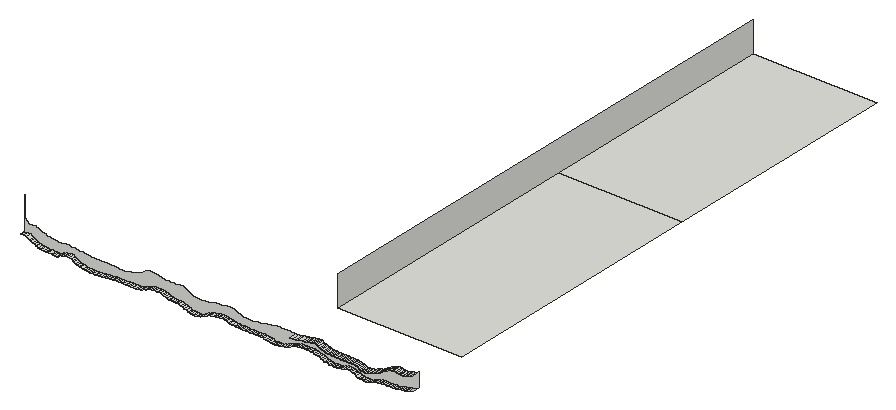
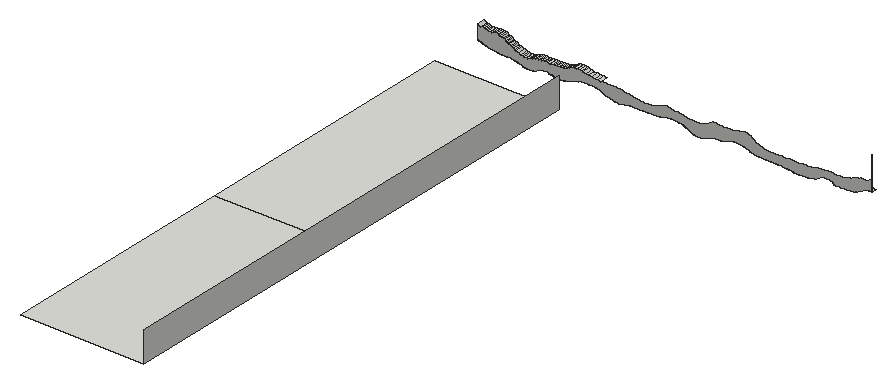
# SketchUp Ruby script. Lengths in inches.
U = 1.inch
M = Sketchup.active_model
def pt(a) = Geom::Point3d.new(a.map { |v| v * U })
def face(e, loops, mat)
  f = e.add_face(loops[0].map { |a| pt(a) })
  loops[1..].each { |l| e.add_face(l.map { |a| pt(a) }).erase! }
  f.material = f.back_material = mat if mat
  f
end
# faces: each face lists its corners as indices into pts; further lists are holes
def faces(e, pts, list, mat = nil) = list.each { |f| face(e, (f[0].is_a?(Array) ? f : [f]).map { |l| l.map { |i| pts[i] } }, mat) }
# xy, xz, yz: faces in a plane at the given z, y or x. An outline is a flat list of corners, or four numbers for a rectangle; further outlines are holes
def ring(l) = l.size == 4 ? [[l[0], l[1]], [l[2], l[1]], [l[2], l[3]], [l[0], l[3]]] : l.each_slice(2).to_a
def flat(e, list, mat, &to3) = list.each { |f| face(e, (f[0].is_a?(Array) ? f : [f]).map { |l| ring(l).map { |u, v| to3.(u, v) } }, mat) }
def xy(e, z, list, mat = nil) = flat(e, list, mat) { |x, y| [x, y, z] }
def xz(e, y, list, mat = nil) = flat(e, list, mat) { |x, z| [x, y, z] }
def yz(e, x, list, mat = nil) = flat(e, list, mat) { |y, z| [x, y, z] }
def lines(e, pts, list) = list.each { |a, b| e.add_line(pt(pts[a]), pt(pts[b])) }
# prism: a flat outline (further loops are holes) pulled along v
def prism(e, loops, v, mat = nil)
  f = face(e, loops, mat); d = Geom::Vector3d.new(v.map { |x| x * U })
  f.pushpull(f.normal.samedirection?(d) ? d.length : -d.length)
end
def box(e, o, s, mat = nil) = prism(e, [[o, [o[0] + s[0], o[1], o[2]], [o[0] + s[0], o[1] + s[1], o[2]], [o[0], o[1] + s[1], o[2]]]], [0, 0, s[2]], mat)
def at(x, y, z, deg = 0) = Geom::Transformation.translation(pt([x, y, z])) * Geom::Transformation.rotation(ORIGIN, Z_AXIS, deg.degrees)
def axes(o, x, y, z) = Geom::Transformation.new([*x, 0, *y, 0, *z, 0, *pt(o).to_a, 1])
def part(name) = M.definitions.add(name)
# library, detail: a bought-in or finely detailed component or shape, given as its bounding box
def library(name, o, s) = part(name).tap { |d| box(d.entities, o, s) }
def detail(e, o, s) = box(e.add_group.entities, o, s)
def put(e, d, t, mat = nil) = e.add_instance(d, t).tap { |i| i.material = mat if mat }
def group(e, t, mat = nil) = e.add_group.tap { |g| g.transformation = t; g.material = mat if mat }.entities
root = M.entities
xy(root,237.65,[[1160.83,566.68,1161.52,568.68],[1161.52,566.68,1162.14,568.68]])
xy(root,238.18,[[1254.78,566.68,1255.46,568.68]])
xy(root,238.33,[[1169.93,566.68,1170.48,568.68],[1170.48,566.68,1171.16,568.68]])
xy(root,238.34,[[1171.84,566.68,1172.77,568.68],[1172.77,566.68,1173.26,568.68],[1173.26,566.68,1174.02,568.68],[1174.02,566.68,1174.65,568.68],[1174.65,566.68,1175.4,568.68],
  [1175.4,566.68,1176.02,568.68],[1176.02,566.68,1176.79,568.68],[1176.79,566.68,1177.41,568.68]])
xy(root,238.62,[[1221.31,566.68,1222.08,568.68],[1222.08,566.68,1222.71,568.68],[1222.71,566.68,1223.47,568.68],[1223.47,566.68,1224.09,568.68],[1224.09,566.68,1224.94,568.68],
  [1224.94,566.68,1225.58,568.68],[1225.58,566.68,1226.2,568.68]])
xy(root,238.625,[[1219.89,566.68,1220.75,568.68]])
xy(root,238.89,[[1275.7,566.68,1276.38,568.68]])
xy(root,238.9,[[1277.14,566.68,1277.76,568.68],[1277.76,566.68,1278.53,568.68]])
xy(root,240.43,[[1243.98,566.68,1244.55,568.68]])
xy(root,241.52,[[1131.53,566.68,1131.59,568.68]])
xy(root,242.28,[[1261.8,565.74,1262.3125,568.68]])
xy(root,242.3,[[1260.04,565.74,1260.71,568.68]])
xy(root,242.33,[[1257.63,565.74,1258.21,568.68]])
xy(root,242.625,[[1237.14,589.83,1285.6,697.21],[1237.14,697.21,1285.6,792.52]])
xz(root,568.68,[[1200.45,236.98,1199.84,237.01,1199.15,237.04,1198.39,237.11,1197.7,237.2,1197.17,237.33,1196.5,237.68,1195.5625,237.96,1195,238.28,1194.22,238.43,1193.44,238.78,1192.77,238.79,1192.23,238.8,1191.47,238.83,1190.72,238.875,1190.15,238.94,1189.57,239.04,1188.91,239.29,1188.33,239.53,1187.8,239.7,1187.11,239.92,1186.48,240.11,1185.7,240.27,1185.08,240.25,1184.375,240.23,1183.61,240.19,1182.9375,240.12,1182.28,240.03,1181.64,239.85,1181.09,239.52,1180.53,239.35,1179.94,239.18,1179.43,238.86,1178.74,238.72,1177.92,238.59,1177.41,238.34,1171.84,238.34,1171.16,238.33,1169.93,238.33,1169.21,238.32,1168.36,238.3,1167.73,238.28,1166.98,238.26,1166.35,238.15,1165.59,238.13,1165.04,238.1,1164.1875,237.98,1163.57,237.94,1162.81,237.89,1162.14,237.65,1160.83,237.65,1160.14,237.66,1159.39,237.67,1158.79,237.68,1158.18,237.71,1157.47,237.76,1156.78,237.82,1156.12,237.9,1155.18,238.21,1154.71,238.31,1153.8,238.43,1153.15,238.74,1152.57,239.11,1151.99,239.38,1151.53,239.71,1150.83,240.11,1150.14,240.09,1149.48,240.05,1148.89,239.99,1148.16,239.88,1147.61,239.69,1147.03,239.55,1146.47,238.9375,1145.94,238.77,1145.2,238.79,1144.33,238.8,1143.82,238.82,1142.78,238.92,1142.09,238.93,1141.39,238.94,1140.69,238.97,1140.01,239.03,1139.32,239.09,1138.54,239.19,1138.03,239.52,1137.47,239.64,1137.02,239.86,1136.23,240.2,1135.63,240.59,1135.09,240.85,1134.07,241.55,1132.8,241.69,1131.59,241.52,1131.59,246.2,1133.16,244.96,1134.55,244.9375,1135.8,244.92,1136.02,244.61,1136.58,244.54,1137.34,244.41,1138.01,244.11,1138.53,243.95,1139.19,243.79,1139.71,243.48,1140.35,243.3,1140.9375,243.14,1141.42,243.06,1142.14,242.85,1142.72,242.78,1143.53,242.73,1144.07,242.68,1144.74,242.51,1145.26,242.46,1145.8,242.58,1146.43,242.57,1147.06,242.81,1147.63,242.86,1148.19,242.89,1148.83,242.92,1149.26,242.625,1149.87,242.65,1150.42,242.62,1151.05,242.58,1151.61,242.57,1152.25,242.48,1152.91,242.38,1153.57,242.34,1154.24,242.24,1155.41,241.96,1156.18,241.89,1157,241.83,1157.6,241.78,1158.37,241.75,1158.82,241.74,1159.37,241.72,1160.63,241.7,1161.36,241.69,1162.03,241.68,1162.62,241.68,1163.11,241.67,1163.8125,241.74,1164.38,241.75,1166.38,241.75,1166.87,241.67,1167.4,241.66,1168.01,241.57,1168.55,241.53,1169.17,241.51,1169.72,241.49,1170.42,241.48,1171.08,241.47,1171.65,241.46,1172.36,241.6,1173.09,241.85,1173.76,241.91,1174.66,242.1,1175.43,242.46,1176.13,242.78,1176.9,242.97,1177.43,243.23,1177.83,243.48,1178.35,243.72,1178.6875,244.12,1179.16,244.39,1179.64,244.73,1180.125,244.87,1180.71,244.95,1181.39,245.01,1182.04,244.81,1182.61,244.7,1183.09,244.67,1183.7,244.55,1184.24,244.51,1184.7,244.25,1185.45,244.11,1186.01,244.04,1186.63,243.99,1187.35,243.95,1187.85,243.93,1188.54,243.91,1189.11,243.89,1189.81,243.88,1190.46,243.94,1191.1,243.95,1191.66,244.1,1192.29,244.13,1192.77,244.15,1193.29,244.17,1193.81,244.18,1194.41,243.8,1194.95,243.43,1195.56,243.09,1195.95,242.875,1196.45,242.68,1197.04,242.51,1197.55,242.21,1198.15,242.11,1198.83,241.96,1199.39,241.89,1199.85,241.85,1200.37,241.8125,1200.88,241.79,1201.46,241.78,1202.13,241.91,1202.6,241.93,1203.27,242.09,1204.04,242.2,1204.54,242.24,1205.15,242.42,1205.7,242.47,1206.45,242.71,1207.09,242.78,1207.57,242.82,1208.26,242.85,1208.96,242.87,1209.51,243.02,1210.13,243.05,1210.68,243.29,1211.36,243.35,1211.91,243.39,1212.51,243.42,1213.28,243.14,1213.85,242.9375,1214.4,242.65,1215.02,242.39,1215.78,242.14,1216.42,241.89,1216.91,241.78,1217.96,241.63,1218.73,241.56,1219.33,241.51,1219.78,241.48,1220.3,241.46,1221.17,241.51,1221.89,241.59,1222.83,241.82,1223.61,241.87,1224.375,241.98,1224.99,242.02,1225.64,242.19,1226.34,242.38,1226.83,242.4375,1227.35,242.48,1228.01,242.58,1228.54,242.61,1229.125,242.77,1229.58,242.95,1230.14,243.01,1230.65,243.05,1231.22,243.08,1231.875,243.09,1234.03,243.09,1234.6,243.08,1235.1875,243.07,1235.77,243.07,1236.43,243.0625,1237.04,243.05,1237.72,243.05,1238.99,243.1,1240.16,243.17,1241.3,243.4,1242.5625,243.52,1243.69,243.71,1244.59,243.99,1245.29,244.08,1245.99,244.21,1246.57,244.27,1247.11,244.3,1247.78,244.39,1248.375,244.19,1248.75,243.88,1249.23,243.59,1249.78,243.33,1250.33,243.22,1250.82,242.92,1251.3,242.75,1251.86,242.6,1252.42,242.52,1252.98,242.47,1253.5625,242.43,1254.14,242.4,1254.72,242.39,1255.3,242.37,1255.88,242.36,1256.47,242.35,1257.63,242.33,1258.21,242.33,1258.93,242.32,1259.4,242.3125,1260.04,242.3,1260.71,242.3,1261.16,242.29,1261.8,242.28,1262.3125,242.28,1262.94,242.2,1263.52,241.97,1264.09,241.84,1264.6,241.57,1265.02,241.33,1265.49,241.24,1266.02,241.17,1266.49,241.12,1267.09,241.09,1267.66,241.14,1268.3,241.35,1268.89,241.46,1269.83,241.85,1270.83,242.23,1271.39,242.42,1272.11,242.61,1272.625,242.91,1273,243.14,1273.54,243.52,1274.02,243.71,1274.35,244.02,1274.79,244.21,1275.38,244.57,1275.85,244.76,1276.47,245.125,1276.97,245.32,1277.45,245.41,1278,245.48,1278.49,245.59,1279.02,245.55,1279.63,245.35,1280.12,245.31,1280.67,245.27,1281.23,245.24,1281.79,245.22,1282.35,245.34,1282.98,245.42,1283.5625,245.52,1283.94,245.76,1284.41,245.9,1285.6,246.43,1285.6,240.89,1283.77,240.1,1283.21,239.96,1282.6875,239.81,1282,239.53,1281.45,239.49,1280.73,239.42,1279.93,239.28,1279.16,239.15,1278.53,238.9,1277.14,238.9,1276.38,238.89,1275.7,238.89,1275.02,238.88,1274.48,238.875,1273.72,238.86,1272.98,238.83,1272.41,238.8,1271.83,238.74,1271.17,238.6,1270.6,238.51,1270.07,238.33,1269.38,238.08,1268.7,237.84,1268.01,237.5625,1267.41,237.47,1266.73,237.4,1266,237.42,1265.43,237.45,1264.84,237.51,1264.24,237.59,1263.7,237.71,1262.87,238,1262.16,238.33,1261.61,238.57,1261.11,238.86,1260.59,238.96,1259.9,239.02,1259.22,239.125,1258.48,239.04,1257.91,238.66,1257.32,238.61,1256.66,238.55,1256.14,238.27,1255.46,238.18,1254.78,238.18,1254.11,238.11,1253.58,238.15,1252.76,238.19,1252.1875,238.26,1251.62,238.48,1250.96,238.56,1250.39,238.67,1249.87,239.01,1249.1875,239.18,1248.5625,239.5,1247.8,239.65,1247.1875,239.8,1246.43,239.96,1245.78,240.23,1245.2,240.27,1244.55,240.43,1243.98,240.43,1243.4,240.42,1242.875,240.41,1242.18,240.4,1241.49,240.37,1240.8,240.33,1240.12,240.27,1239.44,240.17,1238.82,239.97,1238.17,239.75,1237.43,239.375,1236.64,239.08,1235.76,238.72,1235.01,238.46,1233.79,238.14,1232.67,237.88,1232.02,237.87,1231.15,237.74,1230.44,237.79,1229.67,237.86,1229.04,238.15,1228.27,238.19,1227.65,238.25,1226.89,238.45,1226.2,238.62,1221.31,238.62,1220.75,238.625,1219.89,238.625,1219.2,238.63,1218.58,238.64,1217.8,238.65,1217.13,238.66,1216.44,238.6875,1215.77,238.73,1215.29,238.78,1214.41,238.93,1213.64,239.07,1213.09,239.16,1212.24,239.44,1211.57,239.56,1210.96,239.72,1210.23,239.7,1209.67,239.69,1209.08,239.65,1208.46,239.6,1207.97,239.54,1207.16,239.31,1206.16,239.22,1205.58,239.12,1204.9375,238.76,1204.3,238.51,1203.74,238.375,1203.3,238.02,1202.6,237.74,1201.98,237.43,1201.13,237.22],[1131.53,241.52,1131.59,254.5]])
yz(root,1237.14,[[589.83,242.625,792.52,254.5]])
p = [[1198.39,568.68,237.11],[1199.15,568.68,237.04],[1199.15,566.68,237.04],[1198.39,566.68,237.11],[1199.84,568.68,237.01],[1199.84,566.68,237.01],
  [1200.45,568.68,236.98],[1200.45,566.68,236.98],[1201.13,568.68,237.22],[1201.13,566.68,237.22],[1197.7,568.68,237.2],[1197.7,566.68,237.2],
  [1197.17,568.68,237.33],[1197.17,566.68,237.33],[1201.98,568.68,237.43],[1201.98,566.68,237.43],[1196.5,568.68,237.68],[1196.5,566.68,237.68],
  [1202.6,568.68,237.74],[1202.6,566.68,237.74],[1265.43,568.68,237.45],[1266,568.68,237.42],[1266,566.68,237.42],[1265.43,566.68,237.45],
  [1266.73,568.68,237.4],[1266.73,566.68,237.4],[1267.41,568.68,237.47],[1267.41,566.68,237.47],[1264.24,568.68,237.59],[1264.84,568.68,237.51],
  [1264.84,566.68,237.51],[1264.24,566.68,237.59],[1268.01,568.68,237.5625],[1268.01,566.68,237.5625],[1162.14,568.68,237.65],[1162.81,568.68,237.89],
  [1162.81,566.68,237.89],[1162.14,566.68,237.65],[1263.7,568.68,237.71],[1263.7,566.68,237.71],[1268.7,568.68,237.84],[1268.7,566.68,237.84],
  [1157.47,568.68,237.76],[1158.18,568.68,237.71],[1158.18,566.68,237.71],[1157.47,566.68,237.76],[1158.79,568.68,237.68],[1158.79,566.68,237.68],
  [1159.39,568.68,237.67],[1159.39,566.68,237.67],[1160.14,568.68,237.66],[1160.14,566.68,237.66],[1160.83,568.68,237.65],[1160.83,566.68,237.65],
  [1195.5625,568.68,237.96],[1195.5625,566.68,237.96],[1203.3,568.68,238.02],[1203.3,566.68,238.02],[1230.44,568.68,237.79],[1231.15,568.68,237.74],
  [1231.15,566.68,237.74],[1230.44,566.68,237.79],[1232.02,568.68,237.87],[1232.02,566.68,237.87],[1262.87,568.68,238],[1262.87,566.68,238],
  [1156.12,568.68,237.9],[1156.78,568.68,237.82],[1156.78,566.68,237.82],[1156.12,566.68,237.9],[1229.67,568.68,237.86],[1229.67,566.68,237.86],
  [1269.38,568.68,238.08],[1269.38,566.68,238.08],[1155.18,568.68,238.21],[1155.18,566.68,238.21],[1163.57,568.68,237.94],[1163.57,566.68,237.94],
  [1164.1875,568.68,237.98],[1164.1875,566.68,237.98],[1229.04,568.68,238.15],[1229.04,566.68,238.15],[1232.67,568.68,237.88],[1232.67,566.68,237.88],
  [1233.79,568.68,238.14],[1233.79,566.68,238.14],[1165.04,568.68,238.1],[1165.04,566.68,238.1],[1195,568.68,238.28],[1195,566.68,238.28],
  [1203.74,568.68,238.375],[1203.74,566.68,238.375],[1262.16,568.68,238.33],[1262.16,566.68,238.33],[1165.59,568.68,238.13],[1165.59,566.68,238.13],
  [1166.35,568.68,238.15],[1166.35,566.68,238.15],[1228.27,568.68,238.19],[1228.27,566.68,238.19],[1235.01,568.68,238.46],[1235.01,566.68,238.46],
  [1252.76,568.68,238.19],[1253.58,568.68,238.15],[1253.58,566.68,238.15],[1252.76,566.68,238.19],[1254.11,568.68,238.11],[1254.11,566.68,238.11],
  [1254.78,568.68,238.18],[1254.78,566.68,238.18],[1270.07,568.68,238.33],[1270.07,566.68,238.33],[1154.71,568.68,238.31],[1154.71,566.68,238.31],
  [1166.98,568.68,238.26],[1166.98,566.68,238.26],[1227.65,568.68,238.25],[1227.65,566.68,238.25],[1252.1875,568.68,238.26],[1252.1875,566.68,238.26],
  [1255.46,568.68,238.18],[1256.14,568.68,238.27],[1256.14,566.68,238.27],[1255.46,566.68,238.18],[1153.8,568.68,238.43],[1153.8,566.68,238.43],
  [1167.73,568.68,238.28],[1167.73,566.68,238.28],[1168.36,568.68,238.3],[1168.36,566.68,238.3],[1169.21,568.68,238.32],[1169.21,566.68,238.32],
  [1169.93,568.68,238.33],[1169.93,566.68,238.33],[1171.16,568.68,238.33],[1171.84,568.68,238.34],[1171.84,566.68,238.34],[1171.16,566.68,238.33],
  [1177.41,568.68,238.34],[1177.92,568.68,238.59],[1177.92,566.68,238.59],[1177.41,566.68,238.34],[1194.22,568.68,238.43],[1194.22,566.68,238.43],
  [1226.89,568.68,238.45],[1226.89,566.68,238.45],[1251.62,568.68,238.48],[1251.62,566.68,238.48],[1256.66,568.68,238.55],[1256.66,566.68,238.55],
  [1261.61,568.68,238.57],[1261.61,566.68,238.57],[1270.6,568.68,238.51],[1270.6,566.68,238.51],[1153.15,568.68,238.74],[1153.15,566.68,238.74],
  [1193.44,568.68,238.78],[1193.44,566.68,238.78],[1204.3,568.68,238.51],[1204.3,566.68,238.51],[1204.9375,568.68,238.76],[1204.9375,566.68,238.76],
  [1226.2,568.68,238.62],[1226.2,566.68,238.62],[1235.76,568.68,238.72],[1235.76,566.68,238.72],[1250.96,568.68,238.56],[1250.96,566.68,238.56],
  [1257.32,568.68,238.61],[1257.32,566.68,238.61],[1271.17,568.68,238.6],[1271.17,566.68,238.6],[1178.74,568.68,238.72],[1178.74,566.68,238.72],
  [1217.13,568.68,238.66],[1217.8,568.68,238.65],[1217.8,566.68,238.65],[1217.13,566.68,238.66],[1218.58,568.68,238.64],[1218.58,566.68,238.64],
  [1219.2,568.68,238.63],[1219.2,566.68,238.63],[1219.89,568.68,238.625],[1219.89,566.68,238.625],[1220.75,568.68,238.625],[1221.31,568.68,238.62],
  [1221.31,566.68,238.62],[1220.75,566.68,238.625],[1250.39,568.68,238.67],[1250.39,566.68,238.67],[1257.91,568.68,238.66],[1257.91,566.68,238.66],
  [1261.11,568.68,238.86],[1261.11,566.68,238.86],[1271.83,568.68,238.74],[1271.83,566.68,238.74],[1152.57,568.68,239.11],[1152.57,566.68,239.11],
  [1179.43,568.68,238.86],[1179.43,566.68,238.86],[1215.29,568.68,238.78],[1215.77,568.68,238.73],[1215.77,566.68,238.73],[1215.29,566.68,238.78],
  [1216.44,568.68,238.6875],[1216.44,566.68,238.6875],[1236.64,568.68,239.08],[1236.64,566.68,239.08],[1249.87,568.68,239.01],[1249.87,566.68,239.01],
  [1258.48,568.68,239.04],[1258.48,566.68,239.04],[1272.41,568.68,238.8],[1272.41,566.68,238.8],[1142.78,568.68,238.92],[1143.82,568.68,238.82],
  [1143.82,566.68,238.82],[1142.78,566.68,238.92],[1144.33,568.68,238.8],[1144.33,566.68,238.8],[1145.2,568.68,238.79],[1145.2,566.68,238.79],
  [1145.94,568.68,238.77],[1145.94,566.68,238.77],[1146.47,568.68,238.9375],[1146.47,566.68,238.9375],[1190.72,568.68,238.875],[1191.47,568.68,238.83],
  [1191.47,566.68,238.83],[1190.72,566.68,238.875],[1192.23,568.68,238.8],[1192.23,566.68,238.8],[1192.77,568.68,238.79],[1192.77,566.68,238.79],
  [1205.58,568.68,239.12],[1205.58,566.68,239.12],[1214.41,568.68,238.93],[1214.41,566.68,238.93],[1272.98,568.68,238.83],[1272.98,566.68,238.83],
  [1273.72,568.68,238.86],[1273.72,566.68,238.86],[1140.69,568.68,238.97],[1141.39,568.68,238.94],[1141.39,566.68,238.94],[1140.69,566.68,238.97],
  [1142.09,568.68,238.93],[1142.09,566.68,238.93],[1147.03,568.68,239.55],[1147.03,566.68,239.55],[1179.94,568.68,239.18],[1179.94,566.68,239.18],
  [1189.57,568.68,239.04],[1190.15,568.68,238.94],[1190.15,566.68,238.94],[1189.57,566.68,239.04],[1213.64,568.68,239.07],[1213.64,566.68,239.07],
  [1260.59,568.68,238.96],[1260.59,566.68,238.96],[1274.48,568.68,238.875],[1274.48,566.68,238.875],[1275.02,568.68,238.88],[1275.02,566.68,238.88],
  [1275.7,568.68,238.89],[1275.7,566.68,238.89],[1276.38,568.68,238.89],[1277.14,568.68,238.9],[1277.14,566.68,238.9],[1276.38,566.68,238.89],
  [1278.53,568.68,238.9],[1279.16,568.68,239.15],[1279.16,566.68,239.15],[1278.53,566.68,238.9],[1139.32,568.68,239.09],[1140.01,568.68,239.03],
  [1140.01,566.68,239.03],[1139.32,566.68,239.09],[1188.91,568.68,239.29],[1188.91,566.68,239.29],[1249.1875,568.68,239.18],[1249.1875,566.68,239.18],
  [1259.22,568.68,239.125],[1259.22,566.68,239.125],[1259.9,568.68,239.02],[1259.9,566.68,239.02],[1138.54,568.68,239.19],[1138.54,566.68,239.19],
  [1151.99,568.68,239.38],[1151.99,566.68,239.38],[1206.16,568.68,239.22],[1206.16,566.68,239.22],[1213.09,568.68,239.16],[1213.09,566.68,239.16],
  [1237.43,568.68,239.375],[1237.43,566.68,239.375],[1138.03,568.68,239.52],[1138.03,566.68,239.52],[1180.53,568.68,239.35],[1180.53,566.68,239.35],
  [1207.16,568.68,239.31],[1207.16,566.68,239.31],[1212.24,568.68,239.44],[1212.24,566.68,239.44],[1248.5625,568.68,239.5],[1248.5625,566.68,239.5],
  [1279.93,568.68,239.28],[1279.93,566.68,239.28],[1188.33,568.68,239.53],[1188.33,566.68,239.53],[1207.97,568.68,239.54],[1207.97,566.68,239.54],
  [1280.73,568.68,239.42],[1280.73,566.68,239.42],[1151.53,568.68,239.71],[1151.53,566.68,239.71],[1181.09,568.68,239.52],[1181.09,566.68,239.52],
  [1211.57,568.68,239.56],[1211.57,566.68,239.56],[1238.17,568.68,239.75],[1238.17,566.68,239.75],[1281.45,568.68,239.49],[1281.45,566.68,239.49],
  [1137.47,568.68,239.64],[1137.47,566.68,239.64],[1181.64,568.68,239.85],[1181.64,566.68,239.85],[1187.8,568.68,239.7],[1187.8,566.68,239.7],
  [1208.46,568.68,239.6],[1208.46,566.68,239.6],[1247.8,568.68,239.65],[1247.8,566.68,239.65],[1282,568.68,239.53],[1282,566.68,239.53],
  [1282.6875,568.68,239.81],[1282.6875,566.68,239.81],[1137.02,568.68,239.86],[1137.02,566.68,239.86],[1147.61,568.68,239.69],[1147.61,566.68,239.69],
  [1209.08,568.68,239.65],[1209.08,566.68,239.65],[1209.67,568.68,239.69],[1209.67,566.68,239.69],[1210.96,568.68,239.72],[1210.96,566.68,239.72],
  [1148.16,568.68,239.88],[1148.16,566.68,239.88],[1150.83,568.68,240.11],[1150.83,566.68,240.11],[1187.11,568.68,239.92],[1187.11,566.68,239.92],
  [1210.23,568.68,239.7],[1210.23,566.68,239.7],[1238.82,568.68,239.97],[1238.82,566.68,239.97],[1247.1875,568.68,239.8],[1247.1875,566.68,239.8],
  [1182.28,568.68,240.03],[1182.28,566.68,240.03],[1246.43,568.68,239.96],[1246.43,566.68,239.96],[1283.21,568.68,239.96],[1283.21,566.68,239.96],
  [1136.23,568.68,240.2],[1136.23,566.68,240.2],[1148.89,568.68,239.99],[1148.89,566.68,239.99],[1186.48,568.68,240.11],[1186.48,566.68,240.11],
  [1149.48,568.68,240.05],[1149.48,566.68,240.05],[1150.14,568.68,240.09],[1150.14,566.68,240.09],[1182.9375,568.68,240.12],[1182.9375,566.68,240.12],
  [1239.44,568.68,240.17],[1239.44,566.68,240.17],[1245.78,568.68,240.23],[1245.78,566.68,240.23],[1283.77,568.68,240.1],[1283.77,566.68,240.1],
  [1183.61,568.68,240.19],[1183.61,566.68,240.19],[1185.7,568.68,240.27],[1185.7,566.68,240.27],[1285.6,568.68,240.89],[1285.6,566.68,240.89],
  [1135.63,568.68,240.59],[1135.63,566.68,240.59],[1184.375,568.68,240.23],[1184.375,566.68,240.23],[1185.08,568.68,240.25],[1185.08,566.68,240.25],
  [1240.12,568.68,240.27],[1240.12,566.68,240.27],[1245.2,568.68,240.27],[1245.2,566.68,240.27],[1240.8,568.68,240.33],[1240.8,566.68,240.33],
  [1241.49,568.68,240.37],[1241.49,566.68,240.37],[1244.55,568.68,240.43],[1244.55,566.68,240.43],[1242.18,568.68,240.4],[1242.18,566.68,240.4],
  [1242.875,568.68,240.41],[1242.875,566.68,240.41],[1243.4,568.68,240.42],[1243.4,566.68,240.42],[1243.98,568.68,240.43],[1243.98,566.68,240.43],
  [1135.09,568.68,240.85],[1135.09,566.68,240.85],[1134.07,568.68,241.55],[1134.07,566.68,241.55],[1266.02,568.68,241.17],[1266.49,568.68,241.12],
  [1266.49,565.74,241.12],[1266.02,565.74,241.17],[1267.09,568.68,241.09],[1267.09,565.74,241.09],[1267.66,568.68,241.14],[1267.66,565.74,241.14],
  [1268.3,568.68,241.35],[1268.3,565.74,241.35],[1265.02,568.68,241.33],[1265.49,568.68,241.24],[1265.49,565.74,241.24],[1265.02,565.74,241.33],
  [1264.6,568.68,241.57],[1264.6,565.74,241.57],[1268.89,568.68,241.46],[1268.89,565.74,241.46],[1269.83,568.68,241.85],[1269.83,565.74,241.85],
  [1131.59,568.68,241.52],[1132.8,568.68,241.69],[1132.8,566.68,241.69],[1131.59,566.68,241.52],[1264.09,568.68,241.84],[1264.09,565.74,241.84],
  [1263.52,568.68,241.97],[1263.52,565.74,241.97],[1270.83,568.68,242.23],[1270.83,565.74,242.23],[1262.94,568.68,242.2],[1262.94,565.74,242.2],
  [1262.3125,568.68,242.28],[1262.3125,565.74,242.28],[1271.39,568.68,242.42],[1271.39,565.74,242.42],[1256.47,568.68,242.35],[1257.05,568.68,242.34],
  [1257.05,565.74,242.34],[1256.47,565.74,242.35],[1257.63,568.68,242.33],[1257.63,565.74,242.33],[1258.21,568.68,242.33],[1258.93,568.68,242.32],
  [1258.93,565.74,242.32],[1258.21,565.74,242.33],[1259.4,568.68,242.3125],[1259.4,565.74,242.3125],[1260.04,568.68,242.3],[1260.04,565.74,242.3],
  [1260.71,568.68,242.3],[1261.16,568.68,242.29],[1261.16,565.74,242.29],[1260.71,565.74,242.3],[1261.8,568.68,242.28],[1261.8,565.74,242.28],
  [1252.98,568.68,242.47],[1253.5625,568.68,242.43],[1253.5625,565.74,242.43],[1252.98,565.74,242.47],[1254.14,568.68,242.4],[1254.14,565.74,242.4],
  [1254.72,568.68,242.39],[1254.72,565.74,242.39],[1255.3,568.68,242.37],[1255.3,565.74,242.37],[1255.88,568.68,242.36],[1255.88,565.74,242.36],
  [1272.11,568.68,242.61],[1272.11,565.74,242.61],[1251.86,568.68,242.6],[1252.42,568.68,242.52],[1252.42,565.74,242.52],[1251.86,565.74,242.6],
  [1251.3,568.68,242.75],[1251.3,565.74,242.75],[1272.625,568.68,242.91],[1272.625,565.74,242.91],[1250.82,568.68,242.92],[1250.82,565.74,242.92],
  [1250.33,568.68,243.22],[1250.33,565.74,243.22],[1273,568.68,243.14],[1273,565.74,243.14],[1237.72,568.68,243.05],[1238.99,568.68,243.1],
  [1238.99,565.74,243.1],[1237.72,565.74,243.05],[1240.16,568.68,243.17],[1240.16,565.74,243.17],[1273.54,568.68,243.52],[1273.54,565.74,243.52],
  [1241.3,568.68,243.4],[1241.3,565.74,243.4],[1249.78,568.68,243.33],[1249.78,565.74,243.33],[1249.23,568.68,243.59],[1249.23,565.74,243.59],
  [1242.5625,568.68,243.52],[1242.5625,565.74,243.52],[1243.69,568.68,243.71],[1243.69,565.74,243.71],[1274.02,568.68,243.71],[1274.02,565.74,243.71],
  [1248.75,568.68,243.88],[1248.75,565.74,243.88],[1244.59,568.68,243.99],[1244.59,565.74,243.99],[1274.35,568.68,244.02],[1274.35,565.74,244.02],
  [1248.375,568.68,244.19],[1248.375,565.74,244.19],[1245.29,568.68,244.08],[1245.29,565.74,244.08],[1274.79,568.68,244.21],[1274.79,565.74,244.21],
  [1245.99,568.68,244.21],[1245.99,565.74,244.21],[1246.57,568.68,244.27],[1246.57,565.74,244.27],[1247.78,568.68,244.39],[1247.78,565.74,244.39],
  [1275.38,568.68,244.57],[1275.38,565.74,244.57],[1247.11,568.68,244.3],[1247.11,565.74,244.3],[1275.85,568.68,244.76],[1275.85,565.74,244.76],
  [1276.47,568.68,245.125],[1276.47,565.74,245.125],[1276.97,568.68,245.32],[1276.97,565.74,245.32],[1280.67,568.68,245.27],[1281.23,568.68,245.24],
  [1281.23,565.74,245.24],[1280.67,565.74,245.27],[1281.79,568.68,245.22],[1281.79,565.74,245.22],[1282.35,568.68,245.34],[1282.35,565.74,245.34],
  [1277.45,568.68,245.41],[1277.45,565.74,245.41],[1279.02,568.68,245.55],[1279.63,568.68,245.35],[1279.63,565.74,245.35],[1279.02,565.74,245.55],
  [1280.12,568.68,245.31],[1280.12,565.74,245.31],[1282.98,568.68,245.42],[1282.98,565.74,245.42],[1278,568.68,245.48],[1278,565.74,245.48],
  [1283.5625,568.68,245.52],[1283.5625,565.74,245.52],[1278.49,568.68,245.59],[1278.49,565.74,245.59],[1283.94,568.68,245.76],[1283.94,565.74,245.76],
  [1284.41,568.68,245.9],[1284.41,565.74,245.9],[1285.6,568.68,246.43],[1285.6,565.74,246.43]]
faces(root,p,[[0,1,2,3],[1,4,5,2],[4,6,7,5],[6,8,9,7],[10,0,3,11],[12,10,11,13],[8,14,15,9],[16,12,13,17],
  [14,18,19,15],[20,21,22,23],[21,24,25,22],[24,26,27,25],[28,29,30,31],[29,20,23,30],[26,32,33,27],[34,35,36,37],
  [38,28,31,39],[32,40,41,33],[42,43,44,45],[43,46,47,44],[46,48,49,47],[48,50,51,49],[50,52,53,51],[54,16,17,55],
  [18,56,57,19],[58,59,60,61],[59,62,63,60],[64,38,39,65],[66,67,68,69],[67,42,45,68],[70,58,61,71],[40,72,73,41],
  [74,66,69,75],[35,76,77,36],[76,78,79,77],[80,70,71,81],[62,82,83,63],[82,84,85,83],[78,86,87,79],[88,54,55,89],
  [56,90,91,57],[92,64,65,93],[86,94,95,87],[94,96,97,95],[98,80,81,99],[84,100,101,85],[102,103,104,105],[103,106,107,104],
  [106,108,109,107],[72,110,111,73],[112,74,75,113],[96,114,115,97],[116,98,99,117],[118,102,105,119],[120,121,122,123],[124,112,113,125],
  [114,126,127,115],[126,128,129,127],[128,130,131,129],[130,132,133,131],[134,135,136,137],[138,139,140,141],[142,88,89,143],[144,116,117,145],
  [146,118,119,147],[121,148,149,122],[150,92,93,151],[110,152,153,111],[154,124,125,155],[156,142,143,157],[90,158,159,91],[158,160,161,159],
  [162,144,145,163],[100,164,165,101],[166,146,147,167],[148,168,169,149],[152,170,171,153],[139,172,173,140],[174,175,176,177],[175,178,179,176],
  [178,180,181,179],[180,182,183,181],[184,185,186,187],[188,166,167,189],[168,190,191,169],[192,150,151,193],[170,194,195,171],[196,154,155,197],
  [172,198,199,173],[200,201,202,203],[201,204,205,202],[204,174,177,205],[164,206,207,165],[208,188,189,209],[190,210,211,191],[194,212,213,195],
  [214,215,216,217],[215,218,219,216],[218,220,221,219],[220,222,223,221],[222,224,225,223],[226,227,228,229],[227,230,231,228],[230,232,233,231],
  [232,156,157,233],[160,234,235,161],[236,200,203,237],[212,238,239,213],[238,240,241,239],[242,243,244,245],[243,246,247,244],[246,214,217,247],
  [224,248,249,225],[198,250,251,199],[252,253,254,255],[253,226,229,254],[256,236,237,257],[258,192,193,259],[240,260,261,241],[260,262,263,261],
  [262,264,265,263],[266,267,268,269],[270,271,272,273],[274,275,276,277],[275,242,245,276],[278,252,255,279],[280,208,209,281],[210,282,283,211],
  [282,284,285,283],[284,258,259,285],[286,274,277,287],[288,196,197,289],[234,290,291,235],[292,256,257,293],[206,294,295,207],[296,286,287,297],
  [250,298,299,251],[290,300,301,291],[302,292,293,303],[304,280,281,305],[271,306,307,272],[308,278,279,309],[300,310,311,301],[306,312,313,307],
  [314,288,289,315],[298,316,317,299],[318,302,303,319],[294,320,321,295],[312,322,323,313],[324,296,297,325],[316,326,327,317],[328,308,309,329],
  [310,330,331,311],[332,304,305,333],[322,334,335,323],[334,336,337,335],[338,324,325,339],[248,340,341,249],[330,342,343,331],[342,344,345,343],
  [346,318,319,347],[340,348,349,341],[350,314,315,351],[352,328,329,353],[344,354,355,345],[354,346,347,355],[320,356,357,321],[358,332,333,359],
  [326,360,361,327],[362,358,359,363],[336,364,365,337],[366,338,339,367],[348,368,369,349],[370,352,353,371],[368,372,373,369],[372,374,375,373],
  [360,376,377,361],[356,378,379,357],[380,362,363,381],[364,382,383,365],[374,350,351,375],[376,384,385,377],[386,370,371,387],[382,388,389,383],
  [390,366,367,391],[384,392,393,385],[392,394,395,393],[378,396,397,379],[398,380,381,399],[394,386,387,395],[396,400,401,397],[400,402,403,401],
  [404,398,399,405],[402,406,407,403],[406,408,409,407],[408,410,411,409],[410,412,413,411],[414,390,391,415],[416,414,415,417],[418,419,420,421],
  [419,422,423,420],[422,424,425,423],[424,426,427,425],[428,429,430,431],[429,418,421,430],[432,428,431,433],[426,434,435,427],[434,436,437,435],
  [438,439,440,441],[442,432,433,443],[439,416,417,440],[444,442,443,445],[436,446,447,437],[448,444,445,449],[450,448,449,451],[446,452,453,447],
  [454,455,456,457],[455,458,459,456],[460,461,462,463],[461,464,465,462],[464,466,467,465],[468,469,470,471],[469,472,473,470],[474,475,476,477],
  [475,478,479,476],[478,480,481,479],[480,482,483,481],[482,484,485,483],[484,454,457,485],[452,486,487,453],[488,489,490,491],[489,474,477,490],
  [492,488,491,493],[486,494,495,487],[496,492,493,497],[498,496,497,499],[494,500,501,495],[502,503,504,505],[503,506,507,504],[500,508,509,501],
  [506,510,511,507],[512,498,499,513],[514,512,513,515],[510,516,517,511],[516,518,519,517],[508,520,521,509],[522,514,515,523],[518,524,525,519],
  [520,526,527,521],[528,522,523,529],[524,530,531,525],[526,532,533,527],[530,534,535,531],[534,536,537,535],[538,528,529,539],[532,540,541,533],
  [536,542,543,537],[542,538,539,543],[540,544,545,541],[544,546,547,545],[546,548,549,547],[550,551,552,553],[551,554,555,552],[554,556,557,555],
  [548,558,559,549],[560,561,562,563],[561,564,565,562],[564,550,553,565],[556,566,567,557],[558,568,569,559],[566,570,571,567],[568,572,573,569],
  [570,574,575,571],[572,560,563,573],[574,576,577,575],[576,578,579,577]])
